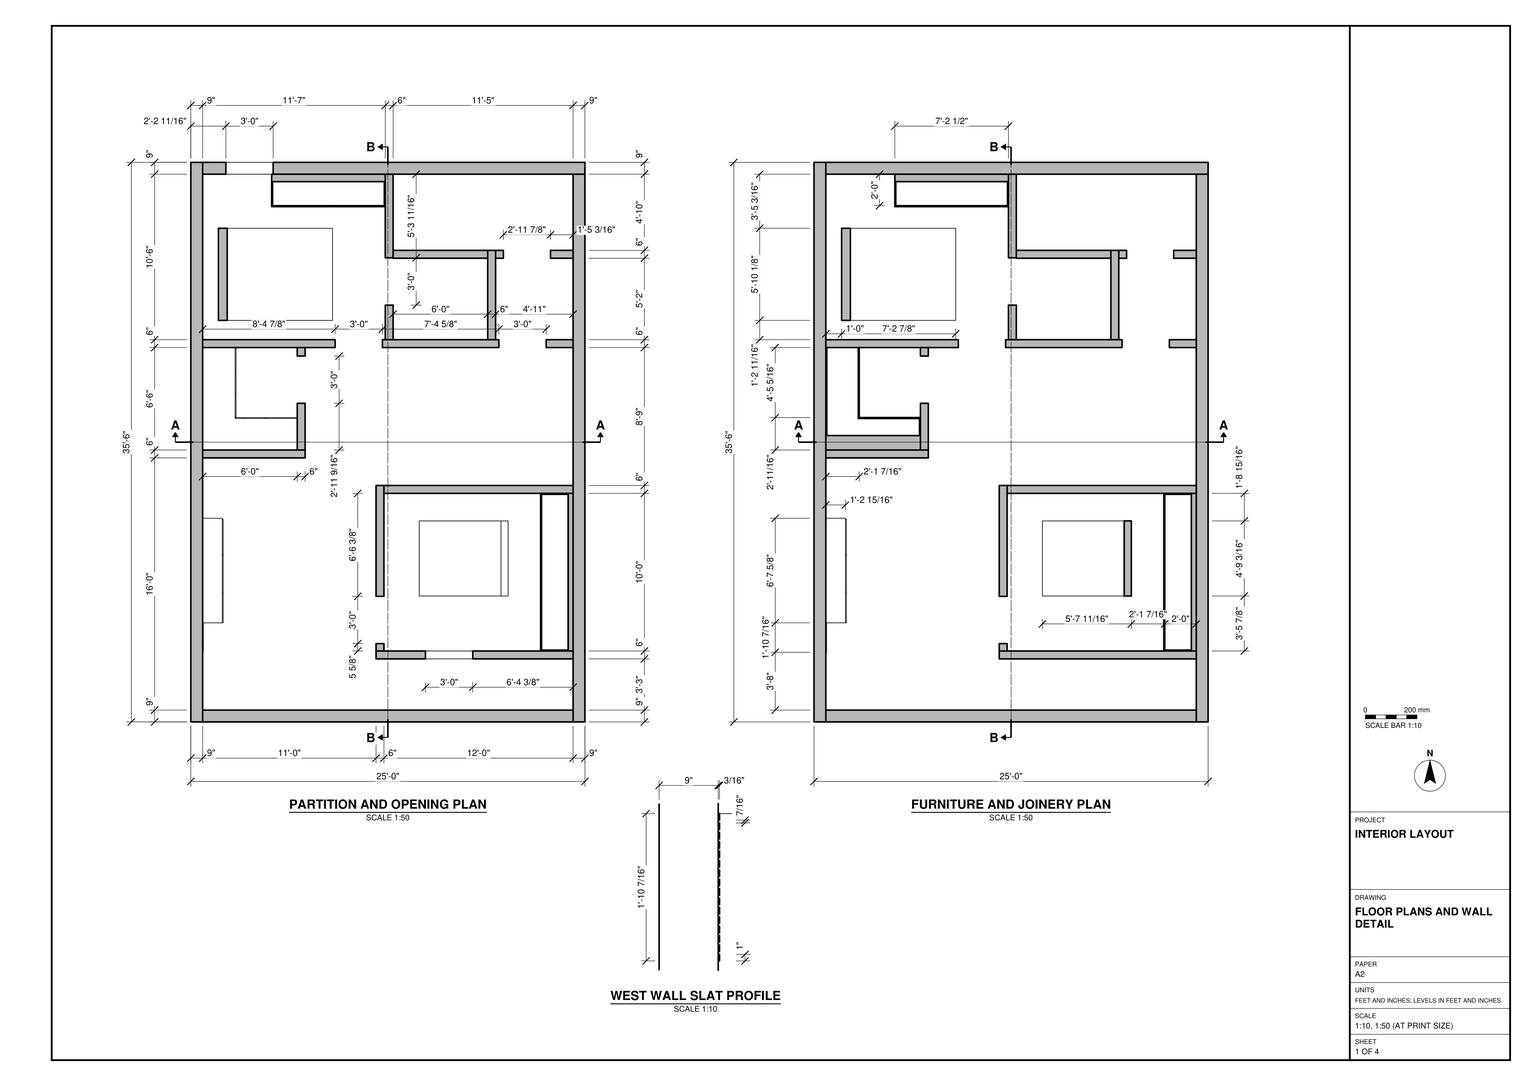
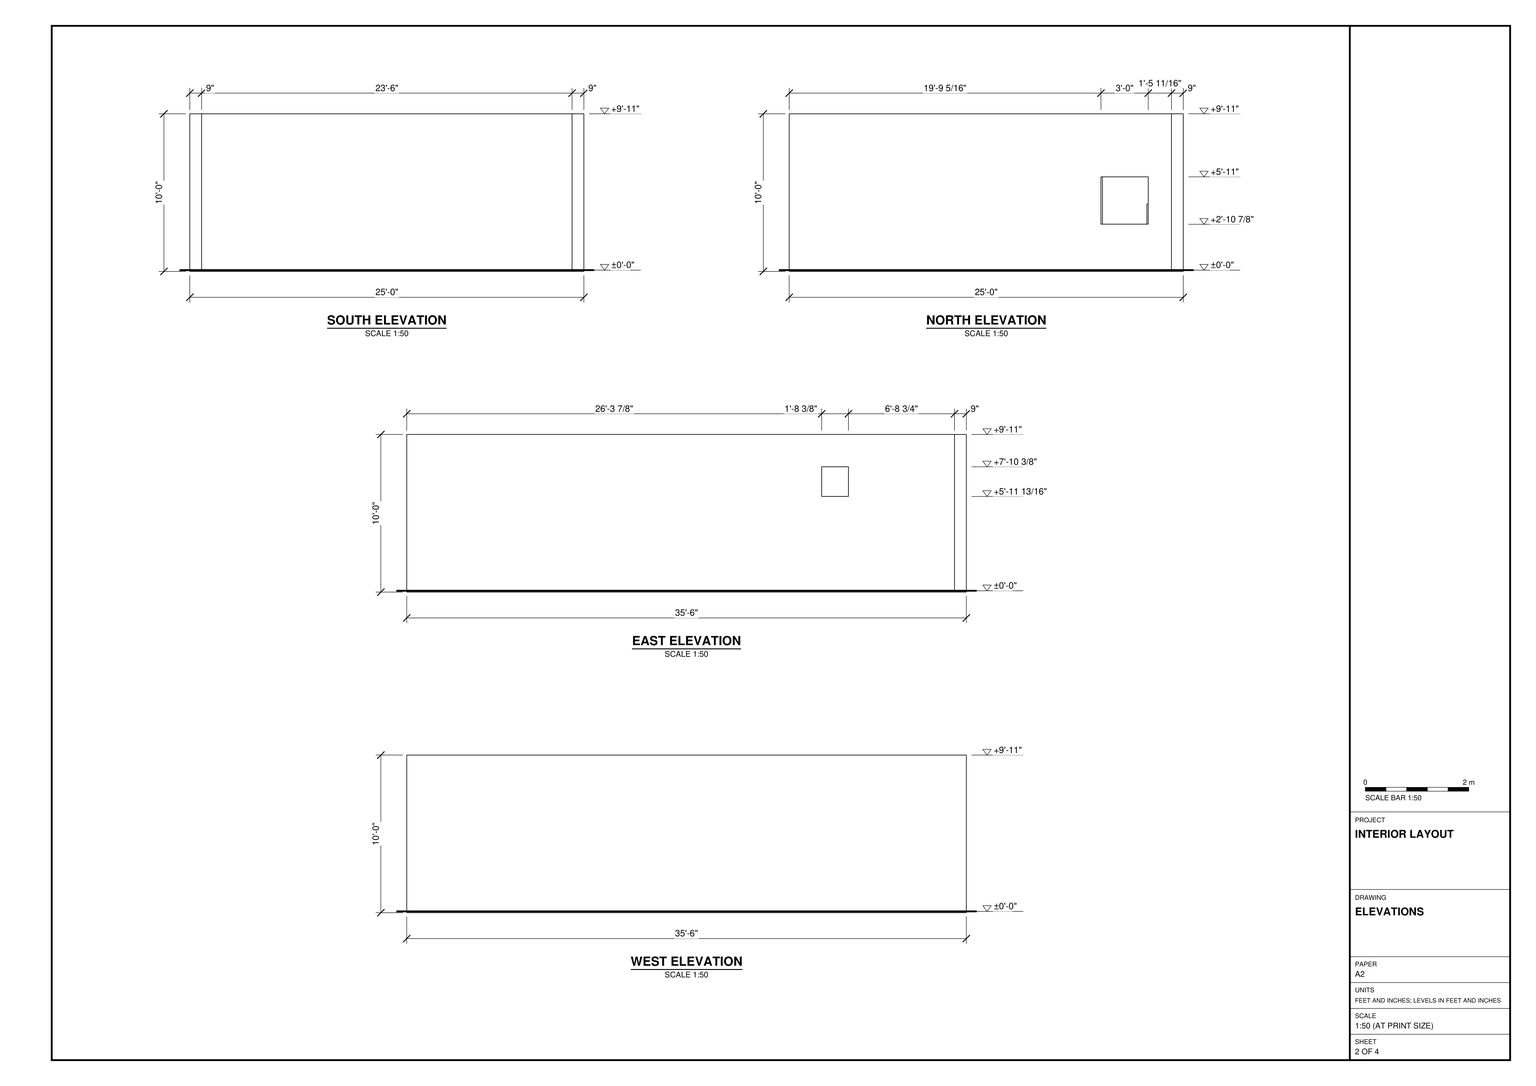
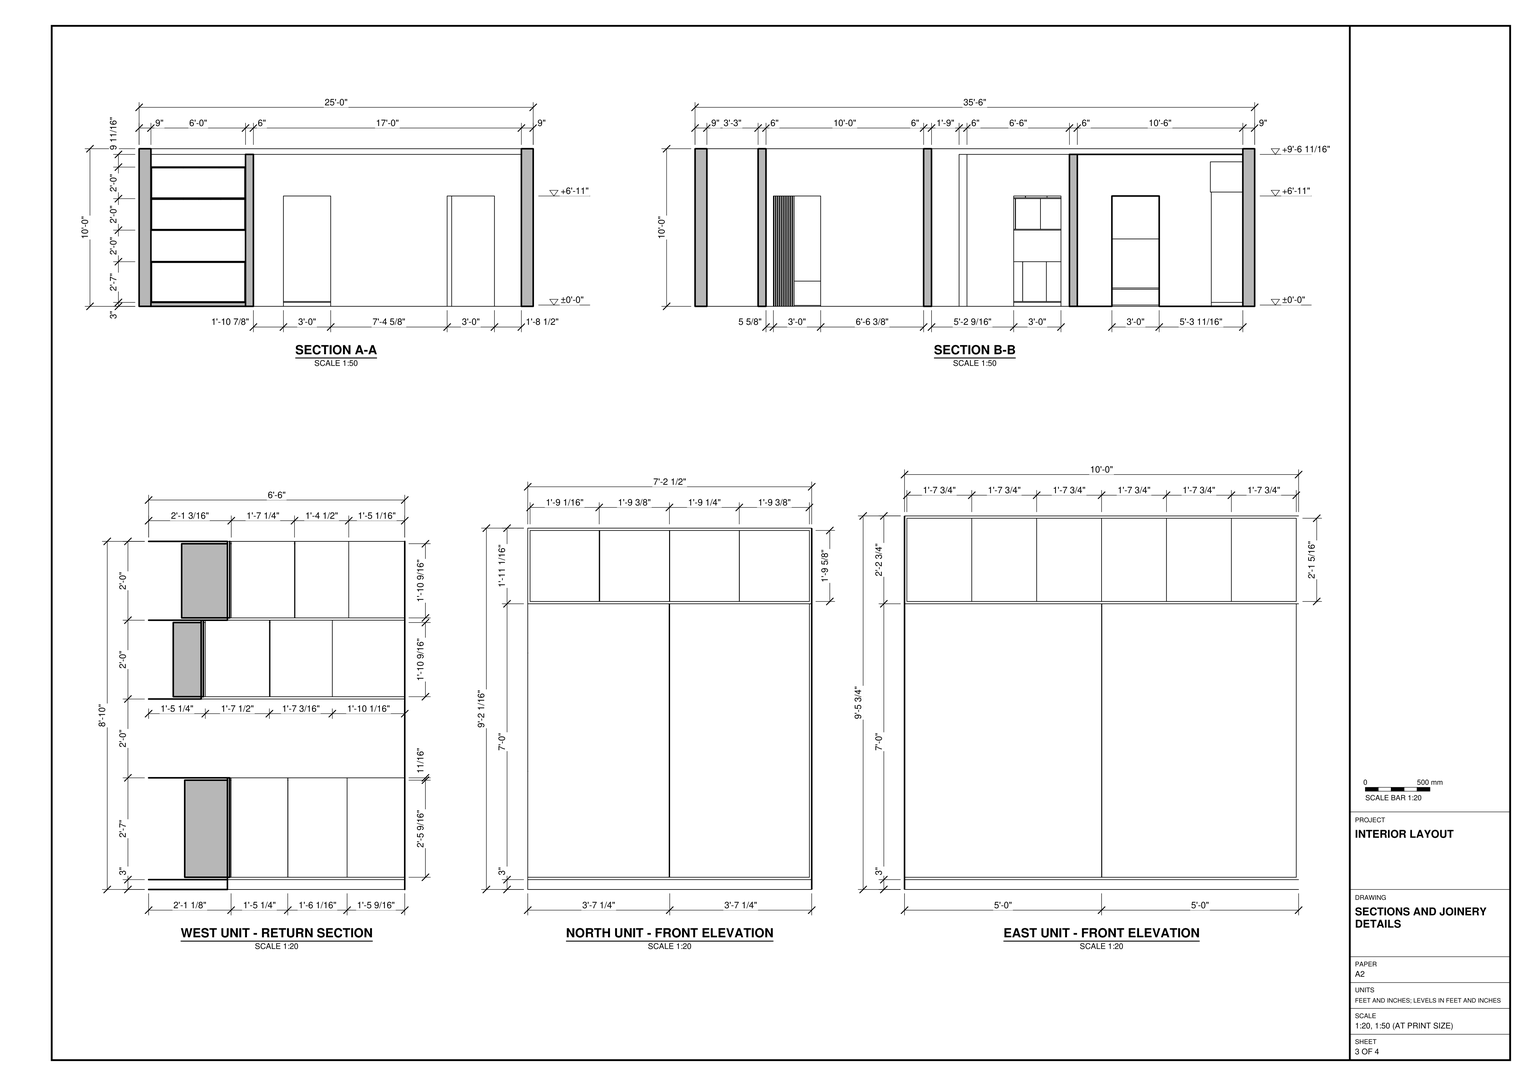
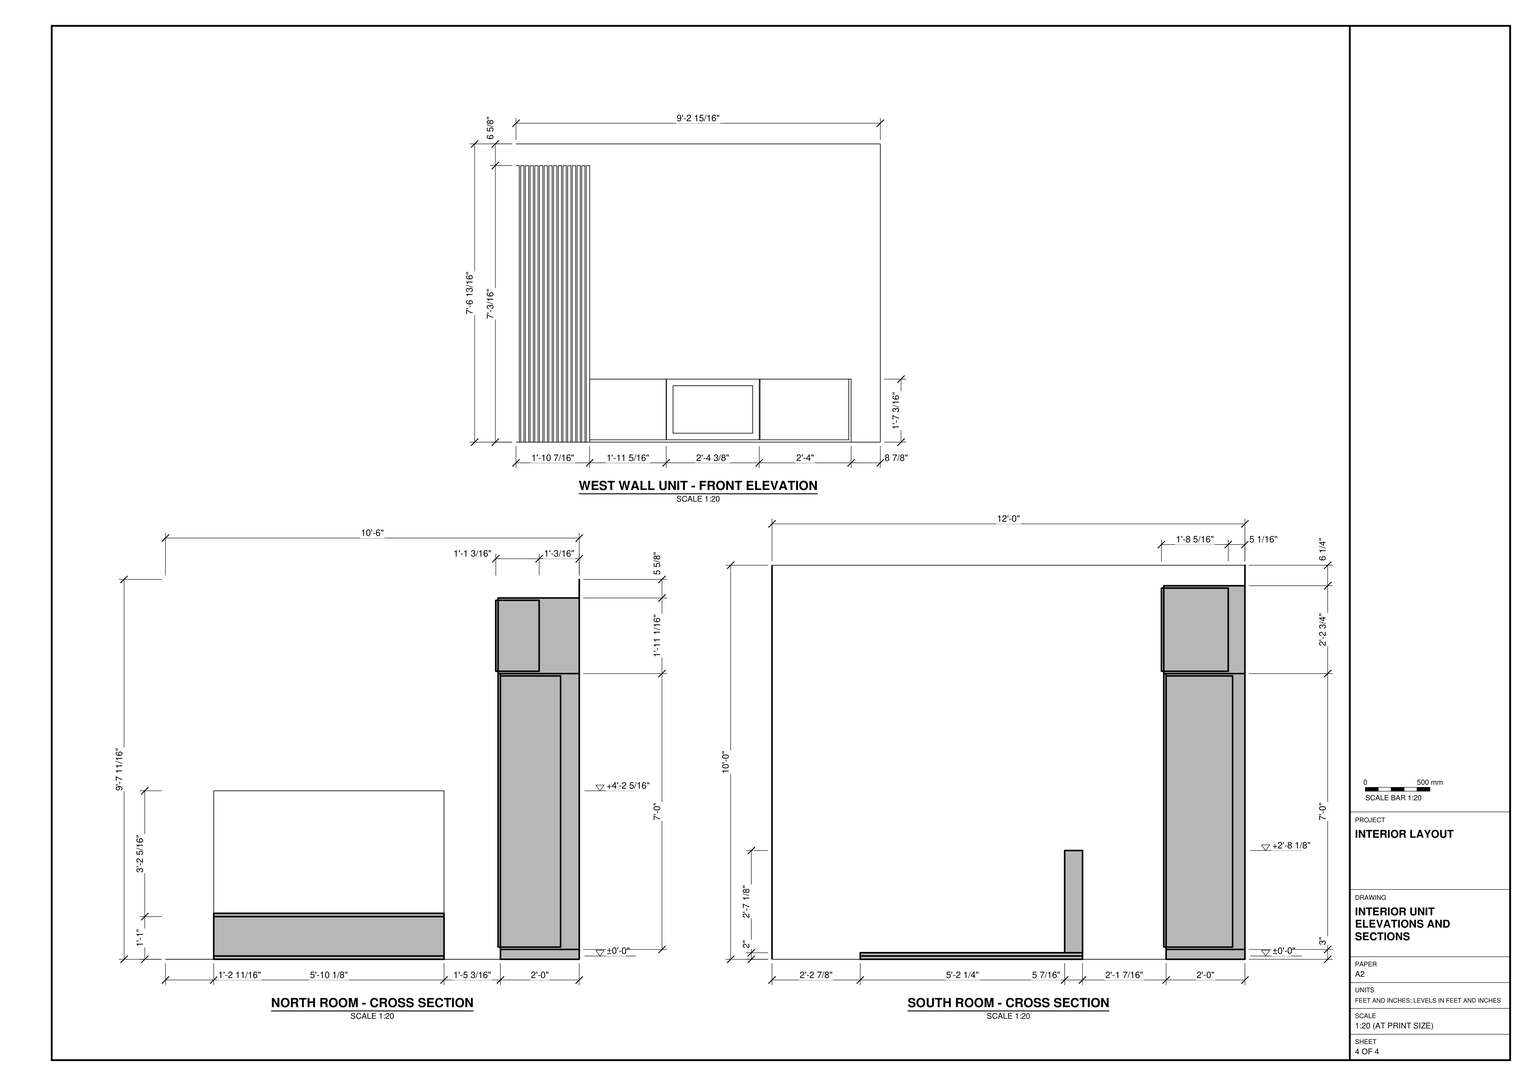
Work in feet and inches in SketchUp. Use task_files/diagram_01.pdf to model the single-storey interior at floor level ±0'-0". The rectangular shell measures 25'-0" east to west by 35'-6" north to south, with an overall height of 10'-0".

Set out the floor, 9" perimeter walls and 6" internal partitions from the partition and opening plan. Form the northwest sleeping area, the smaller partitioned spaces beside it and the southeast room, leaving the central circulation space clear. Use the sections to set the heads of the internal openings. Cut the window opening near the west end of the north wall and the smaller, higher opening in the east wall; leave the south and west exterior elevations uninterrupted.

Position the beds with their headboards at opposite ends as shown on the furniture plan. Model the north and east storage units with their divided upper compartments, tall lower fronts and plinths. Use the return section to build the shelves and dividers of the west unit, and follow the profile detail for the west wall slats.

Keep shell elements and each furniture or joinery piece in separate groups or components, and use components for repeated parts. Any decor or loose items shown may be suitable library components. Save one SketchUp model as output_files/partitioned_interior_with_beds_and_built_in_storage.skp.

# SketchUp Ruby script. Lengths in inches.
U = 1.inch
M = Sketchup.active_model
def pt(a) = Geom::Point3d.new(a.map { |v| v * U })
def face(e, loops, mat)
  f = e.add_face(loops[0].map { |a| pt(a) })
  loops[1..].each { |l| e.add_face(l.map { |a| pt(a) }).erase! }
  f.material = f.back_material = mat if mat
  f
end
# faces: each face lists its corners as indices into pts; further lists are holes
def faces(e, pts, list, mat = nil) = list.each { |f| face(e, (f[0].is_a?(Array) ? f : [f]).map { |l| l.map { |i| pts[i] } }, mat) }
# xy, xz, yz: faces in a plane at the given z, y or x. An outline is a flat list of corners, or four numbers for a rectangle; further outlines are holes
def ring(l) = l.size == 4 ? [[l[0], l[1]], [l[2], l[1]], [l[2], l[3]], [l[0], l[3]]] : l.each_slice(2).to_a
def flat(e, list, mat, &to3) = list.each { |f| face(e, (f[0].is_a?(Array) ? f : [f]).map { |l| ring(l).map { |u, v| to3.(u, v) } }, mat) }
def xy(e, z, list, mat = nil) = flat(e, list, mat) { |x, y| [x, y, z] }
def xz(e, y, list, mat = nil) = flat(e, list, mat) { |x, z| [x, y, z] }
def yz(e, x, list, mat = nil) = flat(e, list, mat) { |y, z| [x, y, z] }
def lines(e, pts, list) = list.each { |a, b| e.add_line(pt(pts[a]), pt(pts[b])) }
# prism: a flat outline (further loops are holes) pulled along v
def prism(e, loops, v, mat = nil)
  f = face(e, loops, mat); d = Geom::Vector3d.new(v.map { |x| x * U })
  f.pushpull(f.normal.samedirection?(d) ? d.length : -d.length)
end
def box(e, o, s, mat = nil) = prism(e, [[o, [o[0] + s[0], o[1], o[2]], [o[0] + s[0], o[1] + s[1], o[2]], [o[0], o[1] + s[1], o[2]]]], [0, 0, s[2]], mat)
def at(x, y, z, deg = 0) = Geom::Transformation.translation(pt([x, y, z])) * Geom::Transformation.rotation(ORIGIN, Z_AXIS, deg.degrees)
def axes(o, x, y, z) = Geom::Transformation.new([*x, 0, *y, 0, *z, 0, *pt(o).to_a, 1])
def part(name) = M.definitions.add(name)
# library, detail: a bought-in or finely detailed component or shape, given as its bounding box
def library(name, o, s) = part(name).tap { |d| box(d.entities, o, s) }
def detail(e, o, s) = box(e.add_group.entities, o, s)
def put(e, d, t, mat = nil) = e.add_instance(d, t).tap { |i| i.material = mat if mat }
def group(e, t, mat = nil) = e.add_group.tap { |g| g.transformation = t; g.material = mat if mat }.entities
root = M.entities
c1 = part("Group\#47")
box(c1.entities,[0,0,0],[0.71,19.76,25.34])
c2 = part("Group\#66")
box(c2.entities,[0,0,0],[0.2,1,84.2])
xy(root,1,[[173.86,95.85,241.55,153.04]])
g1 = group(root,at(0,0,0))
box(g1,[0,0,0],[9,426,120])
g2 = group(root,at(9,417,0))
prism(g2,[[[291,9,0],[0,9,0],[0,9,120],[291,9,120]],[[17.67,9,72],[17.67,9,36],[53.67,9,36],[53.67,9,72]]],[0,-9,0])
g3 = group(root,at(291,0,0))
prism(g3,[[[9,0,0],[9,417,0],[9,417,120],[9,0,120]],[[9,315.875,72.8125],[9,315.875,95.375],[9,336.25,95.375],[9,336.25,72.8125]]],[-9,0,0])
g4 = group(root,at(9,0,0))
box(g4,[0,0,0],[282,9,120])
g5 = group(root,at(9,285,0))
g6 = group(g5,at(0,0,0))
prism(g6,[[[100.86,6,0],[0,6,0],[0,6,115.6875],[282,6,115.6875],[282,6,0],[261.5,6,0],[261.5,6,84],[225.5,6,84],[225.5,6,0],[136.86,6,0],[136.86,6,84],[100.86,6,84]]],[0,-6,0])
g7 = group(root,at(148,291,0))
prism(g7,[[[6,62.32,0],[6,126,0],[6,126,115.6875],[6,0,115.6875],[6,0,0],[6,26.32,0],[6,26.32,84],[6,62.32,84]]],[-6,0,0])
g8 = group(root,at(226,291,0))
box(g8,[0,0,0],[6,68,115.6875])
g9 = group(root,at(154,353,0))
box(g9,[0,0,0],[72,6,115.6875])
g10 = group(root,at(232,353,0))
g11 = group(g10,at(0,0,0))
prism(g11,[[[41.8,0,0],[59,0,0],[59,0,115.6875],[0,0,115.6875],[0,0,0],[5.94,0,0],[5.94,0,84],[41.8,0,84]]],[0,6,0])
g12 = group(root,at(9,201,0))
box(g12,[0,0,0],[78,6,115.6875])
g13 = group(root,at(81,207,0))
prism(g13,[[[0,78,0],[0,71.5625,0],[0,71.5625,84],[0,35.5625,84],[0,35.5625,0],[0,0,0],[0,0,115.6875],[0,78,115.6875]]],[6,0,0])
g14 = group(root,at(141,48,0))
prism(g14,[[[150,6,0],[0,6,0],[0,6,120],[150,6,120]],[[37.625,6,36],[73.625,6,36],[73.625,6,72],[37.625,6,72]]],[0,-6,0])
g15 = group(root,at(141,54,0))
xy(g15,0,[[0,0,6,5.625],[0,41.625,6,126]])
xy(g15,84,[[0,5.625,6,41.625]])
xy(g15,120,[[0,0,6,126]])
xz(g15,0,[[0,0,6,120]])
xz(g15,5.625,[[0,0,6,84]])
xz(g15,41.625,[[0,0,6,84]])
xz(g15,126,[[0,0,6,120]])
yz(g15,0,[[0,0,0,120,126,120,126,0,41.625,0,41.625,84,5.625,84,5.625,0]])
yz(g15,6,[[0,0,5.625,0,5.625,84,41.625,84,41.625,0,120,0,120,120,0,120],[120,0,126,120]])
g16 = group(root,at(147,174,0))
box(g16,[0,0,0],[144,6,120])
g17 = group(root,at(9,207,0))
prism(g17,[[[72,24,0],[72,0,0],[0,0,0],[0,78,0],[24.71,78,0],[24.71,24,0]]],[0,0,3])
g18 = group(root,at(9,207,3))
xy(g18,0,[[0,0,0,78,24.71,78,24.71,24,72,24,72,0]])
xy(g18,0.71,[[0.71,11,71.29,11,71.29,24,24.71,24,24.71,78,0.71,78]])
xy(g18,30.29,[[0.71,11,0.71,78,24.71,78,24.71,24,71.29,24,71.29,11]])
xy(g18,31,[[0,0,72,0,72,24,24.71,24,24.71,78,0,78]])
xz(g18,0,[[0,0,72,31]])
xz(g18,11,[[0.71,0.71,71.29,30.29]])
xz(g18,24,[[24.71,0,24.71,0.71,71.29,0.71,71.29,30.29,24.71,30.29,24.71,31,72,31,72,0]])
xz(g18,78,[[0,0,0,31,24.71,31,24.71,30.29,0.71,30.29,0.71,0.71,24.71,0.71,24.71,0]])
yz(g18,0,[[0,0,78,31]])
yz(g18,0.71,[[11,0.71,78,30.29]])
yz(g18,24.71,[[24,0,78,0.71],[24,30.29,78,31]])
yz(g18,71.29,[[11,0.71,24,30.29]])
yz(g18,72,[[0,0,24,31]])
g19 = group(root,at(9,207,58))
xy(g19,0,[[0,0,0,78,24.71,78,24.71,16,72,16,72,0]])
xy(g19,0.71,[[0.71,7.5,71.29,7.5,71.29,16,24.71,16,24.71,78,0.71,78]])
xy(g19,23.29,[[0.71,7.5,0.71,78,24.71,78,24.71,16,71.29,16,71.29,7.5]])
xy(g19,24,[[0,0,72,0,72,16,24.71,16,24.71,78,0,78]])
xz(g19,0,[[0,0,72,24]])
xz(g19,7.5,[[0.71,0.71,71.29,23.29]])
xz(g19,16,[[24.71,0,24.71,0.71,71.29,0.71,71.29,23.29,24.71,23.29,24.71,24,72,24,72,0]])
xz(g19,78,[[0,0,0,24,24.71,24,24.71,23.29,0.71,23.29,0.71,0.71,24.71,0.71,24.71,0]])
yz(g19,0,[[0,0,78,24]])
yz(g19,0.71,[[7.5,0.71,78,23.29]])
yz(g19,24.71,[[16,0,78,0.71],[16,23.29,78,24]])
yz(g19,71.29,[[7.5,0.71,16,23.29]])
yz(g19,72,[[0,0,16,24]])
g20 = group(root,at(57,231,3.71))
box(g20,[0,0,0],[24,0.71,30.29])
g21 = group(root,at(39.54,231,3.71))
box(g21,[0,0,0],[17.4,0.71,30.29])
g22 = group(root,at(33.71,231,3.71))
box(g22,[0,0,0],[5.76,0.71,30.29])
g23 = group(root,at(33.71,232.11,3.71))
box(g23,[0,0,0],[0.71,17.27,30.29])
g24 = group(root,at(33.71,249.8,3.71))
box(g24,[0,-0.375,0],[0.71,18.02,30.29])
g25 = group(root,at(33.71,267.44,3.71))
box(g25,[0,0,0],[0.71,17.56,30.29])
g26 = group(root,at(62.25,223,58.71))
box(g26,[0,0,0],[18.75,0.71,23.29])
g27 = group(root,at(45.48,223,58.71))
box(g27,[0,0,0],[16.64,0.71,23.29])
g28 = group(root,at(33.71,223,58.71))
box(g28,[0,0,0],[11.77,0.71,23.29])
g29 = group(root,at(33.71,224.28,58.71))
box(g29,[0,0,0],[0.71,19.51,23.29])
g30 = group(root,at(33.71,243.99,58.71))
box(g30,[0,0,0],[0.71,18.95,23.29])
g31 = group(root,at(33.71,262.94,58.71))
box(g31,[0,0,0],[0.71,22.06,23.29])
g32 = group(root,at(9,207,82))
xy(g32,0,[[0,0,0,78,24.71,78,24.71,24,72,24,72,0]])
xy(g32,0.71,[[0.71,10.0625,71.29,10.0625,71.29,24,24.71,24,24.71,78,0.71,78]])
xy(g32,23.29,[[0.71,10.0625,0.71,78,24.71,78,24.71,24,71.29,24,71.29,10.0625]])
xy(g32,24,[[0,0,72,0,72,24,24.71,24,24.71,78,0,78]])
xz(g32,0,[[0,0,72,24]])
xz(g32,10.0625,[[0.71,0.71,71.29,23.29]])
xz(g32,24,[[24.71,0,24.71,0.71,71.29,0.71,71.29,23.29,24.71,23.29,24.71,24,72,24,72,0]])
xz(g32,78,[[0,0,0,24,24.71,24,24.71,23.29,0.71,23.29,0.71,0.71,24.71,0.71,24.71,0]])
yz(g32,0,[[0,0,78,24]])
yz(g32,0.71,[[10.0625,0.71,78,23.29]])
yz(g32,24.71,[[24,0,78,0.71],[24,23.29,78,24]])
yz(g32,71.29,[[10.0625,0.71,24,23.29]])
yz(g32,72,[[0,0,24,24]])
g33 = group(root,at(61.52,393,0))
box(g33,[0,0,0],[86.48,24,3])
g34 = group(root,at(61.52,393,3))
xy(g34,0,[[0,0,86.48,24]])
xy(g34,0.71,[[0.71,0,85.77,18.3125]])
xy(g34,83.29,[[0.71,0,85.77,18.3125]])
xy(g34,84,[[0,0,86.48,24]])
xz(g34,0,[[[0,0,86.48,84],[0.71,0.71,85.77,83.29]]])
xz(g34,18.3125,[[0.71,0.71,85.77,83.29]])
xz(g34,24,[[0,0,86.48,84]])
yz(g34,0,[[0,0,24,84]])
yz(g34,0.71,[[0,0.71,18.3125,83.29]])
yz(g34,85.77,[[0,0.71,18.3125,83.29]])
yz(g34,86.48,[[0,0,24,84]])
g35 = group(root,at(61.52,392.29,3.71))
box(g35,[0,0,0],[43.04,0.71,83.29])
g36 = group(root,at(104.76,392.29,3.71))
box(g36,[0,0,0],[42.53,0.71,83.29])
g37 = group(root,at(61.52,417,87))
xy(g37,0,[[0,-24.71,86.48,0]])
xy(g37,0.71,[[0.71,-24.71,85.77,-12.21]])
xy(g37,22.32,[[0.71,-24.71,85.77,-12.21]])
xy(g37,23.03,[[0,-24.71,86.48,0]])
xz(g37,-24.71,[[[0,0,86.48,23.03],[0.71,0.71,85.77,22.32]]])
xz(g37,-12.21,[[0.71,0.71,85.77,22.32]])
xz(g37,0,[[0,0,86.48,23.03]])
yz(g37,0,[[-24.71,0,0,23.03]])
yz(g37,0.71,[[-24.71,0.71,-12.21,22.32]])
yz(g37,85.77,[[-24.71,0.71,-12.21,22.32]])
yz(g37,86.48,[[-24.71,0,0,23.03]])
g38 = group(root,at(62.23,391.58,87.71))
box(g38,[21.22,0,0],[21.22,0.71,21.62])
p = [[0,0.71,21.62],[21.22,0.71,21.62]]
lines(g38,p,[[0,1]])
g39 = group(root,at(62.23,391.58,87.71))
box(g39,[0,0,0],[21.05,0.71,21.62])
g40 = group(root,at(125.98,391.58,87.71))
box(g40,[0,0,0],[21.31,0.71,21.62])
g41 = group(root,at(104.76,391.58,87.71))
box(g41,[0,0,0],[21.18,0.71,21.62])
g42 = group(root,at(267,54,0))
box(g42,[0,0,0],[24,120,3])
g43 = group(root,at(267,54,3))
xy(g43,0,[[0,0,24,120]])
xy(g43,0.71,[[0,0.71,20.25,119.29]])
xy(g43,83.29,[[0,0.71,20.25,119.29]])
xy(g43,84,[[0,0,24,120]])
xz(g43,0,[[0,0,24,84]])
xz(g43,0.71,[[0,0.71,20.25,83.29]])
xz(g43,119.29,[[0,0.71,20.25,83.29]])
xz(g43,120,[[0,0,24,84]])
yz(g43,0,[[[0,0,120,84],[0.71,0.71,119.29,83.29]]])
yz(g43,20.25,[[0.71,0.71,119.29,83.29]])
yz(g43,24,[[0,0,120,84]])
g44 = group(root,at(266.29,114,3.71))
box(g44,[0,0,0],[0.71,60,83.29])
g45 = group(root,at(266.29,54.71,3.71))
box(g45,[0,0,0],[0.71,59.2,83.29])
g46 = group(root,at(291,54,87))
xy(g46,0,[[-24.71,0,0,120]])
xy(g46,0.71,[[-24.71,0.71,-5.08,119.29]])
xy(g46,26.05,[[-24.71,0.71,-5.08,119.29]])
xy(g46,26.75,[[-24.71,0,0,120]])
xz(g46,0,[[-24.71,0,0,26.75]])
xz(g46,0.71,[[-24.71,0.71,-5.08,26.05]])
xz(g46,119.29,[[-24.71,0.71,-5.08,26.05]])
xz(g46,120,[[-24.71,0,0,26.75]])
yz(g46,-24.71,[[[0,0,120,26.75],[0.71,0.71,119.29,26.05]]])
yz(g46,-5.08,[[0.71,0.71,119.29,26.05]])
yz(g46,0,[[0,0,120,26.75]])
put(root,c1,at(265.58,114,87.71))
put(root,c1,at(265.58,133.76,87.71))
put(root,c1,at(265.58,153.53,87.71))
put(root,c1,at(265.58,54.71,87.71))
put(root,c1,at(265.58,74.47,87.71))
put(root,c1,at(265.58,94.24,87.71))
g47 = group(root,at(21,305.7,0))
box(g47,[0,0,0],[86.875,70.125,1])
g48 = group(root,at(21,305.7,1))
box(g48,[0,0,0],[86.875,70.125,12])
g49 = group(root,at(21,305.7,13))
box(g49,[0,0,0],[86.875,70.125,1])
g50 = group(root,at(21,305.7,14))
box(g50,[0,0,0],[6.6875,70.125,37.3125])
g51 = group(root,at(60.83,231,82.71))
box(g51,[0,0,0],[20.17,0.71,23.29])
g52 = group(root,at(45.71,231,82.71))
box(g52,[0,0,0],[15.06,0.71,23.29])
g53 = group(root,at(33.71,231,82.71))
box(g53,[0,0,0],[12.01,0.71,23.29])
g54 = group(root,at(33.71,232.17,82.71))
box(g54,[0,0,0],[0.71,19.26,23.29])
g55 = group(root,at(33.71,251.57,82.71))
box(g55,[0,0,0],[0.71,16.37,23.29])
g56 = group(root,at(33.71,267.95,82.71))
box(g56,[0,0,0],[0.71,17.05,23.29])
g57 = group(root,at(173.86,95.85,0))
box(g57,[0,0,0],[67.6875,57.1875,1])
g58 = group(root,at(173.86,95.85,1))
box(g58,[0,0,0],[67.6875,57.1875,1])
g59 = group(root,at(236.11,95.85,2))
box(g59,[0,0,0],[5.4375,57.1875,31.125])
g60 = group(root,at(9,53.02,0))
yz(g60,0,[[0,0,110.9375,90.8125]])
g61 = group(root,at(9,75.4375,0))
xy(g61,0,[[0,0,14.9375,79.625]])
xy(g61,0.71,[[5.4375,0.71,14.9375,78.92]])
xy(g61,18.48,[[5.4375,0.71,14.9375,78.92]])
xy(g61,19.1875,[[0,0,14.9375,79.625]])
xz(g61,0,[[0,0,14.9375,19.1875]])
xz(g61,0.71,[[5.4375,0.71,14.9375,18.48]])
xz(g61,78.92,[[5.4375,0.71,14.9375,18.48]])
xz(g61,79.625,[[0,0,14.9375,19.1875]])
yz(g61,0,[[0,0,79.625,19.1875]])
yz(g61,5.4375,[[0.71,0.71,78.92,18.48]])
yz(g61,14.9375,[[[0,0,79.625,19.1875],[0.71,0.71,78.92,18.48]]])
g62 = group(root,at(23.9375,75.4375,0.71))
box(g62,[0,0,0],[0.71,23.3,18.48])
g63 = group(root,at(23.9375,98.84,0.71))
prism(g63,[[[0,0,18.48],[0,28.25,18.48],[0,28.25,0],[0,0,0]],[[0,26.25,16.48],[0,2,16.48],[0,2,2],[0,26.25,2]]],[0.71,0,0])
g64 = group(root,at(23.9375,127.34,0.71))
box(g64,[0,0,0],[0.71,27.01,18.48])
put(root,c2,at(9,53.02,0))
put(root,c2,at(9,54.45,0))
put(root,c2,at(9,55.875,0))
put(root,c2,at(9,57.3,0))
put(root,c2,at(9,58.73,0))
put(root,c2,at(9,60.16,0))
put(root,c2,at(9,61.59,0))
put(root,c2,at(9,63.02,0))
put(root,c2,at(9,64.45,0))
put(root,c2,at(9,65.88,0))
put(root,c2,at(9,67.31,0))
put(root,c2,at(9,68.74,0))
put(root,c2,at(9,70.17,0))
put(root,c2,at(9,71.6,0))
put(root,c2,at(9,73.02,0))
put(root,c2,at(9,74.45,0))
